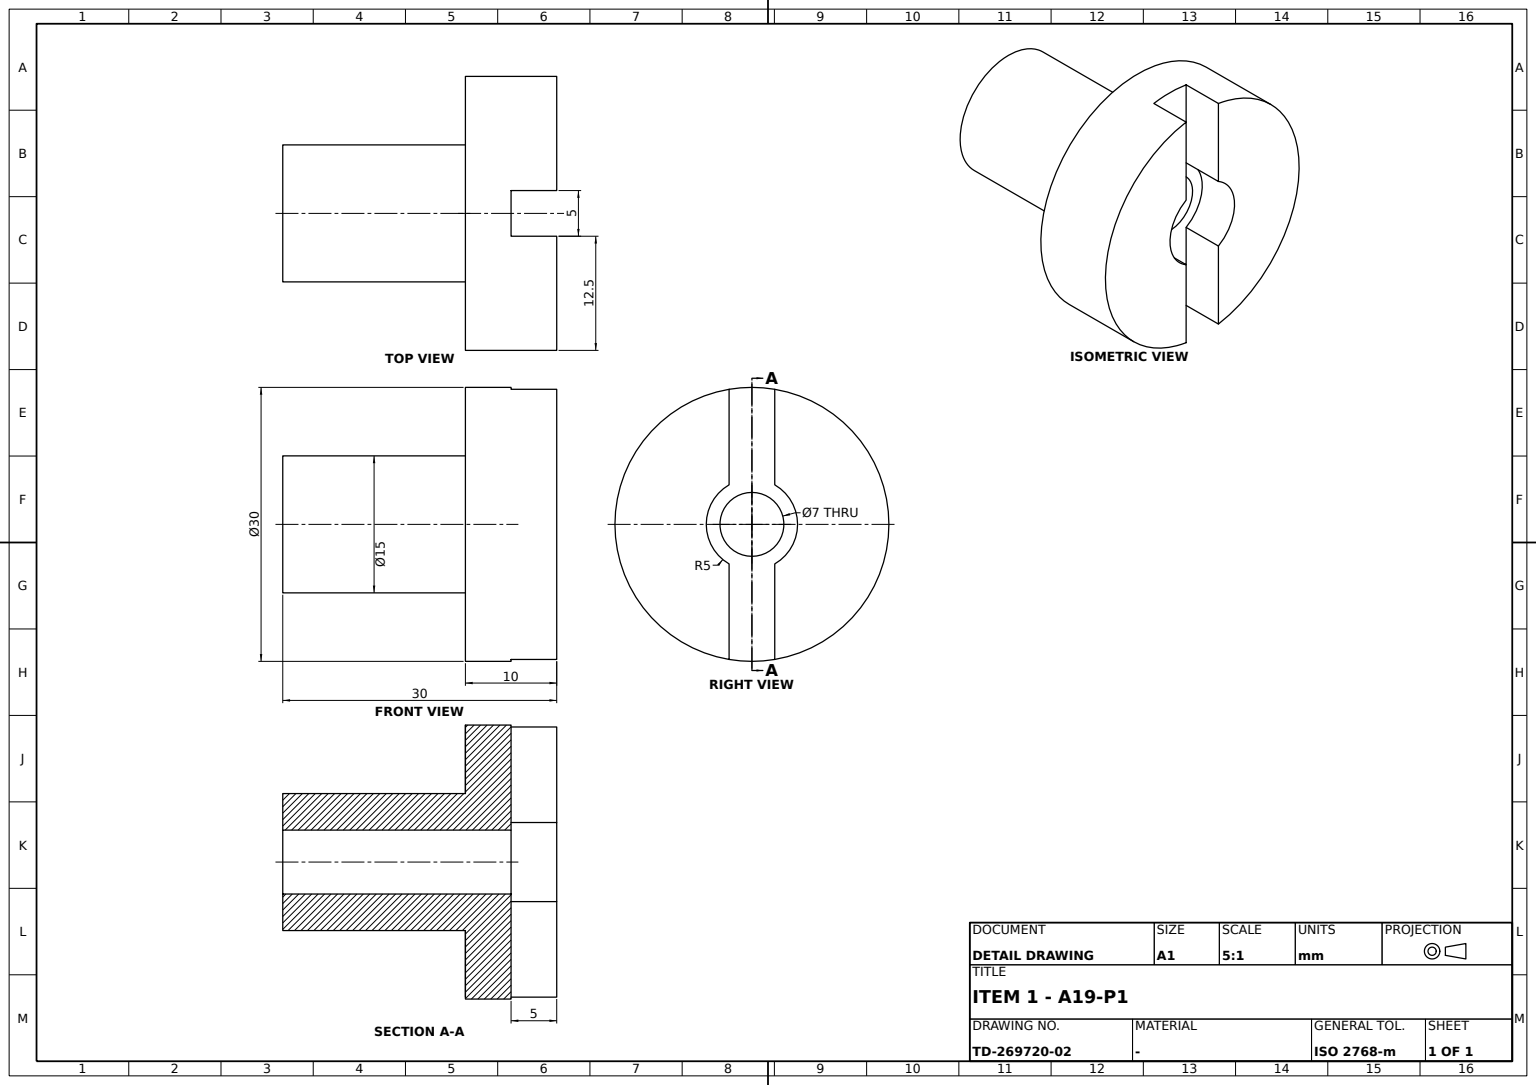
ISO-10303-21;
HEADER;
FILE_DESCRIPTION((''),'2;1');
FILE_NAME('','',(''),(''),'','','');
FILE_SCHEMA(('AUTOMOTIVE_DESIGN'));
ENDSEC;
DATA;
#1=APPLICATION_CONTEXT('');
#2=PRODUCT_CONTEXT('',#1,'mechanical');
#3=PRODUCT('','','',(#2));
#4=PRODUCT_DEFINITION_FORMATION('','',#3);
#5=PRODUCT_DEFINITION_CONTEXT('',#1,'design');
#6=PRODUCT_DEFINITION('','',#4,#5);
#7=PRODUCT_DEFINITION_SHAPE('','',#6);
#8=(LENGTH_UNIT()NAMED_UNIT(*)SI_UNIT(.MILLI.,.METRE.));
#9=(NAMED_UNIT(*)PLANE_ANGLE_UNIT()SI_UNIT($,.RADIAN.));
#10=(NAMED_UNIT(*)SI_UNIT($,.STERADIAN.)SOLID_ANGLE_UNIT());
#11=UNCERTAINTY_MEASURE_WITH_UNIT(LENGTH_MEASURE(0.005),#8,'distance_accuracy_value','');
#12=(GEOMETRIC_REPRESENTATION_CONTEXT(3)GLOBAL_UNCERTAINTY_ASSIGNED_CONTEXT((#11))GLOBAL_UNIT_ASSIGNED_CONTEXT((#8,#9,#10))REPRESENTATION_CONTEXT('',''));
#13=CARTESIAN_POINT('',(0.,-2.5,14.790199));
#14=VERTEX_POINT('',#13);
#15=CARTESIAN_POINT('',(0.,-2.5,-14.790199));
#16=VERTEX_POINT('',#15);
#17=CARTESIAN_POINT('',(0.,0.,0.));
#18=DIRECTION('',(1.,0.,0.));
#19=DIRECTION('',(0.,0.,-1.));
#20=AXIS2_PLACEMENT_3D('',#17,#18,#19);
#21=CIRCLE('',#20,15.);
#22=EDGE_CURVE('',#14,#16,#21,.T.);
#23=ORIENTED_EDGE('',*,*,#22,.T.);
#24=CARTESIAN_POINT('',(0.,-2.5,-4.330127));
#25=VERTEX_POINT('',#24);
#26=CARTESIAN_POINT('',(0.,-2.5,4.330127));
#27=DIRECTION('',(0.,0.,1.));
#28=VECTOR('',#27,1000.);
#29=LINE('',#26,#28);
#30=EDGE_CURVE('',#16,#25,#29,.T.);
#31=ORIENTED_EDGE('',*,*,#30,.T.);
#32=VERTEX_POINT('',#26);
#33=CIRCLE('',#20,5.);
#34=EDGE_CURVE('',#32,#25,#33,.T.);
#35=ORIENTED_EDGE('',*,*,#34,.F.);
#36=EDGE_CURVE('',#32,#14,#29,.T.);
#37=ORIENTED_EDGE('',*,*,#36,.T.);
#38=EDGE_LOOP('',(#23,#31,#35,#37));
#39=FACE_BOUND('',#38,.T.);
#40=DIRECTION('',(0.,1.,0.));
#41=AXIS2_PLACEMENT_3D('',#17,#18,#40);
#42=PLANE('',#41);
#43=ADVANCED_FACE('',(#39),#42,.T.);
#44=CARTESIAN_POINT('',(-30.,0.,7.5));
#45=VERTEX_POINT('',#44);
#46=CARTESIAN_POINT('',(-30.,0.,0.));
#47=DIRECTION('',(-1.,0.,0.));
#48=AXIS2_PLACEMENT_3D('',#46,#47,#27);
#49=CIRCLE('',#48,7.5);
#50=EDGE_CURVE('',#45,#45,#49,.T.);
#51=ORIENTED_EDGE('',*,*,#50,.F.);
#52=EDGE_LOOP('',(#51));
#53=FACE_BOUND('',#52,.T.);
#54=CARTESIAN_POINT('',(-10.,0.,-7.5));
#55=VERTEX_POINT('',#54);
#56=CARTESIAN_POINT('',(-10.,0.,0.));
#57=AXIS2_PLACEMENT_3D('',#56,#18,#19);
#58=CIRCLE('',#57,7.5);
#59=EDGE_CURVE('',#55,#55,#58,.F.);
#60=ORIENTED_EDGE('',*,*,#59,.T.);
#61=EDGE_LOOP('',(#60));
#62=FACE_BOUND('',#61,.T.);
#63=CARTESIAN_POINT('',(-20.,0.,0.));
#64=DIRECTION('',(0.,-1.,0.));
#65=AXIS2_PLACEMENT_3D('',#63,#47,#64);
#66=CYLINDRICAL_SURFACE('',#65,7.5);
#67=ADVANCED_FACE('',(#53,#62),#66,.T.);
#68=CARTESIAN_POINT('',(0.,2.5,14.790199));
#69=VERTEX_POINT('',#68);
#70=CARTESIAN_POINT('',(-5.,2.5,14.790199));
#71=VERTEX_POINT('',#70);
#72=VECTOR('',#18,1000.);
#73=LINE('',#68,#72);
#74=EDGE_CURVE('',#69,#71,#73,.F.);
#75=ORIENTED_EDGE('',*,*,#74,.T.);
#76=CARTESIAN_POINT('',(-5.,2.5,4.330127));
#77=VERTEX_POINT('',#76);
#78=CARTESIAN_POINT('',(-5.,2.5,16.330127));
#79=VECTOR('',#19,1000.);
#80=LINE('',#78,#79);
#81=EDGE_CURVE('',#71,#77,#80,.T.);
#82=ORIENTED_EDGE('',*,*,#81,.T.);
#83=CARTESIAN_POINT('',(0.,2.5,4.330127));
#84=VERTEX_POINT('',#83);
#85=LINE('',#83,#72);
#86=EDGE_CURVE('',#84,#77,#85,.F.);
#87=ORIENTED_EDGE('',*,*,#86,.F.);
#88=CARTESIAN_POINT('',(0.,2.5,16.330127));
#89=LINE('',#88,#79);
#90=EDGE_CURVE('',#69,#84,#89,.T.);
#91=ORIENTED_EDGE('',*,*,#90,.F.);
#92=EDGE_LOOP('',(#75,#82,#87,#91));
#93=FACE_BOUND('',#92,.T.);
#94=AXIS2_PLACEMENT_3D('',#88,#40,#19);
#95=PLANE('',#94);
#96=ADVANCED_FACE('',(#93),#95,.F.);
#97=CARTESIAN_POINT('',(-5.,0.,-3.5));
#98=VERTEX_POINT('',#97);
#99=CARTESIAN_POINT('',(-5.,0.,0.));
#100=AXIS2_PLACEMENT_3D('',#99,#18,#19);
#101=CIRCLE('',#100,3.5);
#102=EDGE_CURVE('',#98,#98,#101,.T.);
#103=ORIENTED_EDGE('',*,*,#102,.F.);
#104=EDGE_LOOP('',(#103));
#105=FACE_BOUND('',#104,.T.);
#106=CARTESIAN_POINT('',(-5.,2.5,-4.330127));
#107=VERTEX_POINT('',#106);
#108=CARTESIAN_POINT('',(-5.,2.5,-14.790199));
#109=VERTEX_POINT('',#108);
#110=EDGE_CURVE('',#107,#109,#80,.T.);
#111=ORIENTED_EDGE('',*,*,#110,.F.);
#112=CIRCLE('',#100,5.);
#113=EDGE_CURVE('',#107,#77,#112,.T.);
#114=ORIENTED_EDGE('',*,*,#113,.T.);
#115=ORIENTED_EDGE('',*,*,#81,.F.);
#116=CARTESIAN_POINT('',(-5.,-2.5,14.790199));
#117=VERTEX_POINT('',#116);
#118=CIRCLE('',#100,15.);
#119=EDGE_CURVE('',#71,#117,#118,.T.);
#120=ORIENTED_EDGE('',*,*,#119,.T.);
#121=CARTESIAN_POINT('',(-5.,-2.5,4.330127));
#122=VERTEX_POINT('',#121);
#123=LINE('',#121,#28);
#124=EDGE_CURVE('',#122,#117,#123,.T.);
#125=ORIENTED_EDGE('',*,*,#124,.F.);
#126=CARTESIAN_POINT('',(-5.,-2.5,-4.330127));
#127=VERTEX_POINT('',#126);
#128=EDGE_CURVE('',#122,#127,#112,.T.);
#129=ORIENTED_EDGE('',*,*,#128,.T.);
#130=CARTESIAN_POINT('',(-5.,-2.5,-14.790199));
#131=VERTEX_POINT('',#130);
#132=EDGE_CURVE('',#131,#127,#123,.T.);
#133=ORIENTED_EDGE('',*,*,#132,.F.);
#134=EDGE_CURVE('',#131,#109,#118,.T.);
#135=ORIENTED_EDGE('',*,*,#134,.T.);
#136=EDGE_LOOP('',(#111,#114,#115,#120,#125,#129,#133,#135));
#137=FACE_BOUND('',#136,.T.);
#138=AXIS2_PLACEMENT_3D('',#99,#18,#40);
#139=PLANE('',#138);
#140=ADVANCED_FACE('',(#105,#137),#139,.T.);
#141=ORIENTED_EDGE('',*,*,#113,.F.);
#142=CARTESIAN_POINT('',(0.,2.5,-4.330127));
#143=VERTEX_POINT('',#142);
#144=LINE('',#142,#72);
#145=EDGE_CURVE('',#143,#107,#144,.F.);
#146=ORIENTED_EDGE('',*,*,#145,.F.);
#147=EDGE_CURVE('',#143,#84,#33,.T.);
#148=ORIENTED_EDGE('',*,*,#147,.T.);
#149=ORIENTED_EDGE('',*,*,#86,.T.);
#150=EDGE_LOOP('',(#141,#146,#148,#149));
#151=FACE_BOUND('',#150,.T.);
#152=CARTESIAN_POINT('',(-2.5,0.,0.));
#153=AXIS2_PLACEMENT_3D('',#152,#18,#40);
#154=CYLINDRICAL_SURFACE('',#153,5.);
#155=ADVANCED_FACE('',(#151),#154,.F.);
#156=ORIENTED_EDGE('',*,*,#128,.F.);
#157=LINE('',#26,#72);
#158=EDGE_CURVE('',#32,#122,#157,.F.);
#159=ORIENTED_EDGE('',*,*,#158,.F.);
#160=ORIENTED_EDGE('',*,*,#34,.T.);
#161=LINE('',#24,#72);
#162=EDGE_CURVE('',#25,#127,#161,.F.);
#163=ORIENTED_EDGE('',*,*,#162,.T.);
#164=EDGE_LOOP('',(#156,#159,#160,#163));
#165=FACE_BOUND('',#164,.T.);
#166=ADVANCED_FACE('',(#165),#154,.F.);
#167=ORIENTED_EDGE('',*,*,#132,.T.);
#168=ORIENTED_EDGE('',*,*,#162,.F.);
#169=ORIENTED_EDGE('',*,*,#30,.F.);
#170=LINE('',#15,#72);
#171=EDGE_CURVE('',#16,#131,#170,.F.);
#172=ORIENTED_EDGE('',*,*,#171,.T.);
#173=EDGE_LOOP('',(#167,#168,#169,#172));
#174=FACE_BOUND('',#173,.T.);
#175=AXIS2_PLACEMENT_3D('',#26,#64,#27);
#176=PLANE('',#175);
#177=ADVANCED_FACE('',(#174),#176,.F.);
#178=LINE('',#13,#72);
#179=EDGE_CURVE('',#14,#117,#178,.F.);
#180=ORIENTED_EDGE('',*,*,#179,.F.);
#181=ORIENTED_EDGE('',*,*,#36,.F.);
#182=ORIENTED_EDGE('',*,*,#158,.T.);
#183=ORIENTED_EDGE('',*,*,#124,.T.);
#184=EDGE_LOOP('',(#180,#181,#182,#183));
#185=FACE_BOUND('',#184,.T.);
#186=ADVANCED_FACE('',(#185),#176,.F.);
#187=CARTESIAN_POINT('',(-10.,0.,-15.));
#188=VERTEX_POINT('',#187);
#189=CIRCLE('',#57,15.);
#190=EDGE_CURVE('',#188,#188,#189,.T.);
#191=ORIENTED_EDGE('',*,*,#190,.T.);
#192=EDGE_LOOP('',(#191));
#193=FACE_BOUND('',#192,.T.);
#194=ORIENTED_EDGE('',*,*,#171,.F.);
#195=ORIENTED_EDGE('',*,*,#22,.F.);
#196=ORIENTED_EDGE('',*,*,#179,.T.);
#197=ORIENTED_EDGE('',*,*,#119,.F.);
#198=ORIENTED_EDGE('',*,*,#74,.F.);
#199=CARTESIAN_POINT('',(0.,2.5,-14.790199));
#200=VERTEX_POINT('',#199);
#201=EDGE_CURVE('',#200,#69,#21,.T.);
#202=ORIENTED_EDGE('',*,*,#201,.F.);
#203=LINE('',#199,#72);
#204=EDGE_CURVE('',#200,#109,#203,.F.);
#205=ORIENTED_EDGE('',*,*,#204,.T.);
#206=ORIENTED_EDGE('',*,*,#134,.F.);
#207=EDGE_LOOP('',(#194,#195,#196,#197,#198,#202,#205,#206));
#208=FACE_BOUND('',#207,.T.);
#209=CYLINDRICAL_SURFACE('',#138,15.);
#210=ADVANCED_FACE('',(#193,#208),#209,.T.);
#211=ORIENTED_EDGE('',*,*,#50,.T.);
#212=EDGE_LOOP('',(#211));
#213=FACE_BOUND('',#212,.T.);
#214=CARTESIAN_POINT('',(-30.,0.,3.5));
#215=VERTEX_POINT('',#214);
#216=CIRCLE('',#48,3.5);
#217=EDGE_CURVE('',#215,#215,#216,.T.);
#218=ORIENTED_EDGE('',*,*,#217,.F.);
#219=EDGE_LOOP('',(#218));
#220=FACE_BOUND('',#219,.T.);
#221=AXIS2_PLACEMENT_3D('',#46,#47,#64);
#222=PLANE('',#221);
#223=ADVANCED_FACE('',(#213,#220),#222,.T.);
#224=ORIENTED_EDGE('',*,*,#102,.T.);
#225=EDGE_LOOP('',(#224));
#226=FACE_BOUND('',#225,.T.);
#227=ORIENTED_EDGE('',*,*,#217,.T.);
#228=EDGE_LOOP('',(#227));
#229=FACE_BOUND('',#228,.T.);
#230=CARTESIAN_POINT('',(-6.5,0.,0.));
#231=AXIS2_PLACEMENT_3D('',#230,#47,#64);
#232=CYLINDRICAL_SURFACE('',#231,3.5);
#233=ADVANCED_FACE('',(#226,#229),#232,.F.);
#234=ORIENTED_EDGE('',*,*,#147,.F.);
#235=EDGE_CURVE('',#143,#200,#89,.T.);
#236=ORIENTED_EDGE('',*,*,#235,.T.);
#237=ORIENTED_EDGE('',*,*,#201,.T.);
#238=ORIENTED_EDGE('',*,*,#90,.T.);
#239=EDGE_LOOP('',(#234,#236,#237,#238));
#240=FACE_BOUND('',#239,.T.);
#241=ADVANCED_FACE('',(#240),#42,.T.);
#242=ORIENTED_EDGE('',*,*,#190,.F.);
#243=EDGE_LOOP('',(#242));
#244=FACE_BOUND('',#243,.T.);
#245=ORIENTED_EDGE('',*,*,#59,.F.);
#246=EDGE_LOOP('',(#245));
#247=FACE_BOUND('',#246,.T.);
#248=AXIS2_PLACEMENT_3D('',#56,#18,#40);
#249=PLANE('',#248);
#250=ADVANCED_FACE('',(#244,#247),#249,.F.);
#251=ORIENTED_EDGE('',*,*,#145,.T.);
#252=ORIENTED_EDGE('',*,*,#110,.T.);
#253=ORIENTED_EDGE('',*,*,#204,.F.);
#254=ORIENTED_EDGE('',*,*,#235,.F.);
#255=EDGE_LOOP('',(#251,#252,#253,#254));
#256=FACE_BOUND('',#255,.T.);
#257=ADVANCED_FACE('',(#256),#95,.F.);
#258=CLOSED_SHELL('',(#43,#67,#96,#140,#155,#166,#177,#186,#210,#223,#233,#241,#250,#257));
#259=MANIFOLD_SOLID_BREP('',#258);
#260=ADVANCED_BREP_SHAPE_REPRESENTATION('',(#259),#12);
#261=SHAPE_DEFINITION_REPRESENTATION(#7,#260);
ENDSEC;
END-ISO-10303-21;
